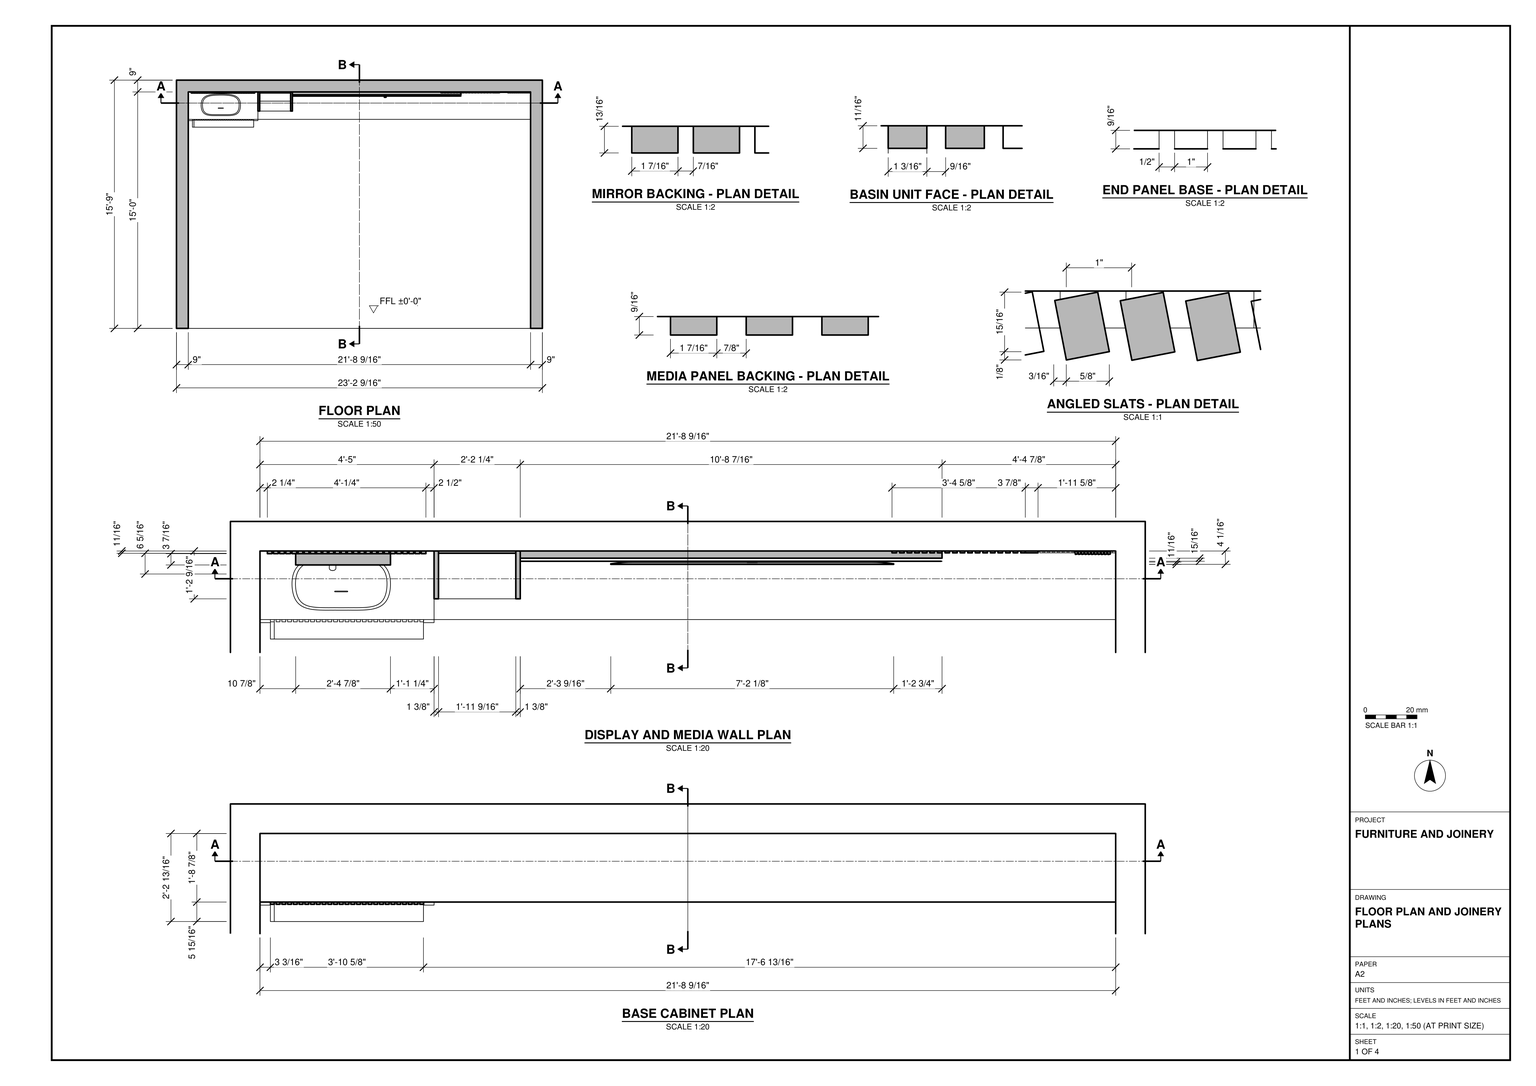
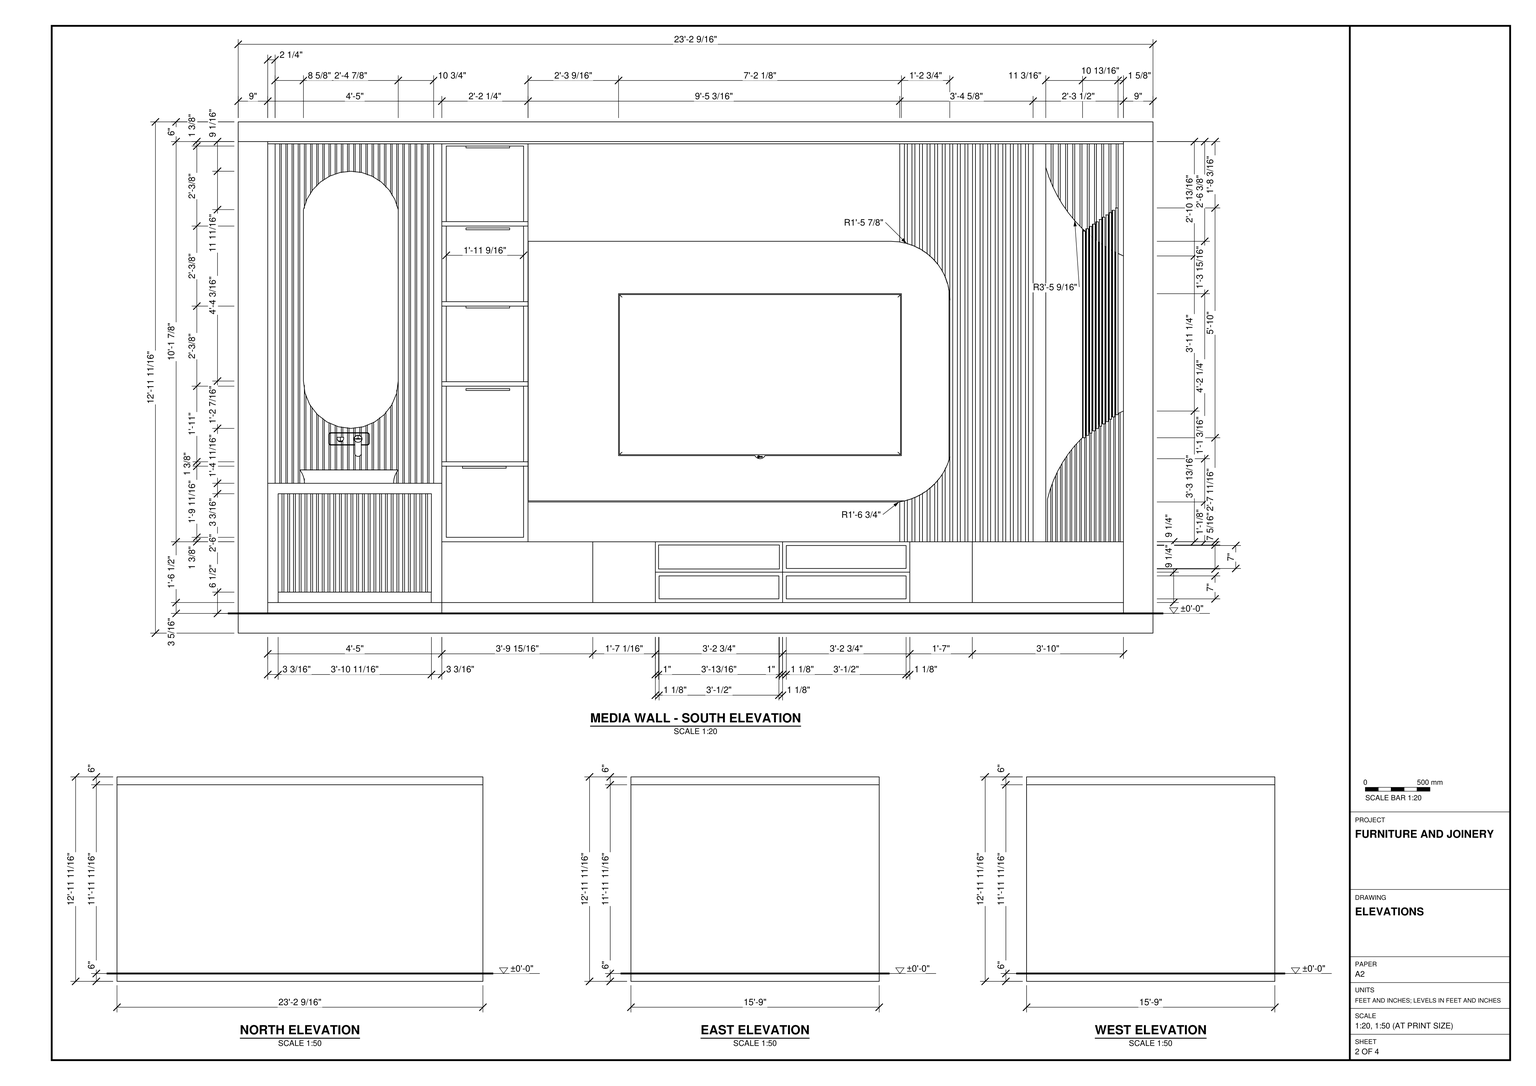
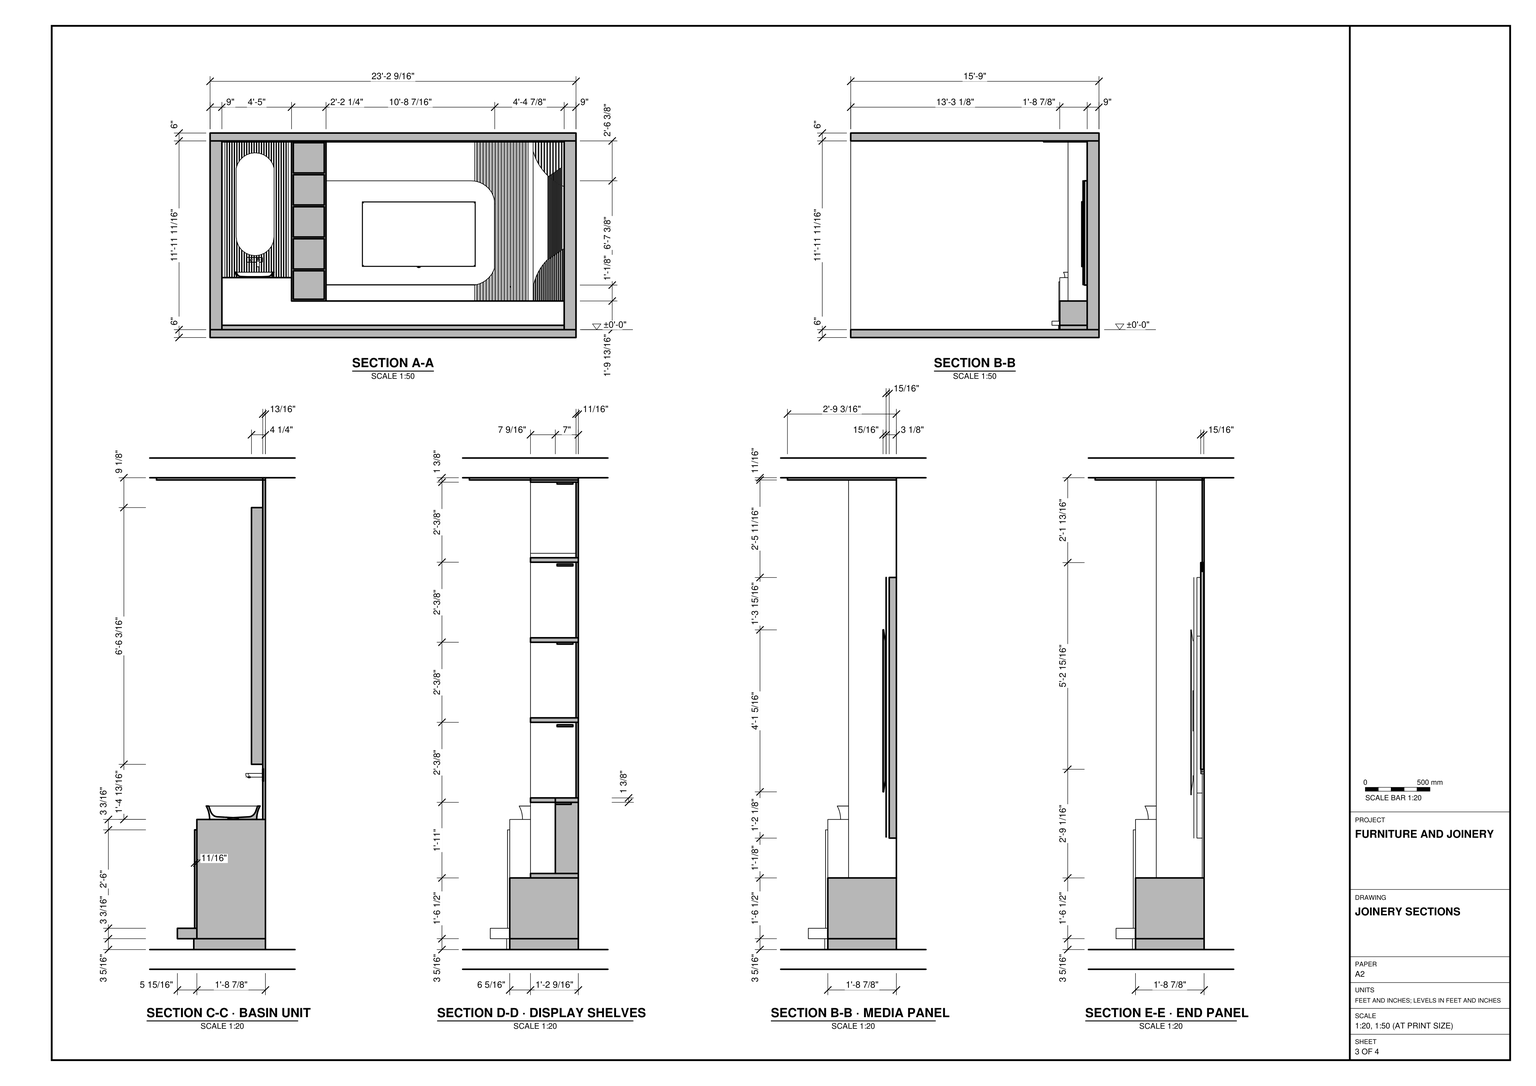
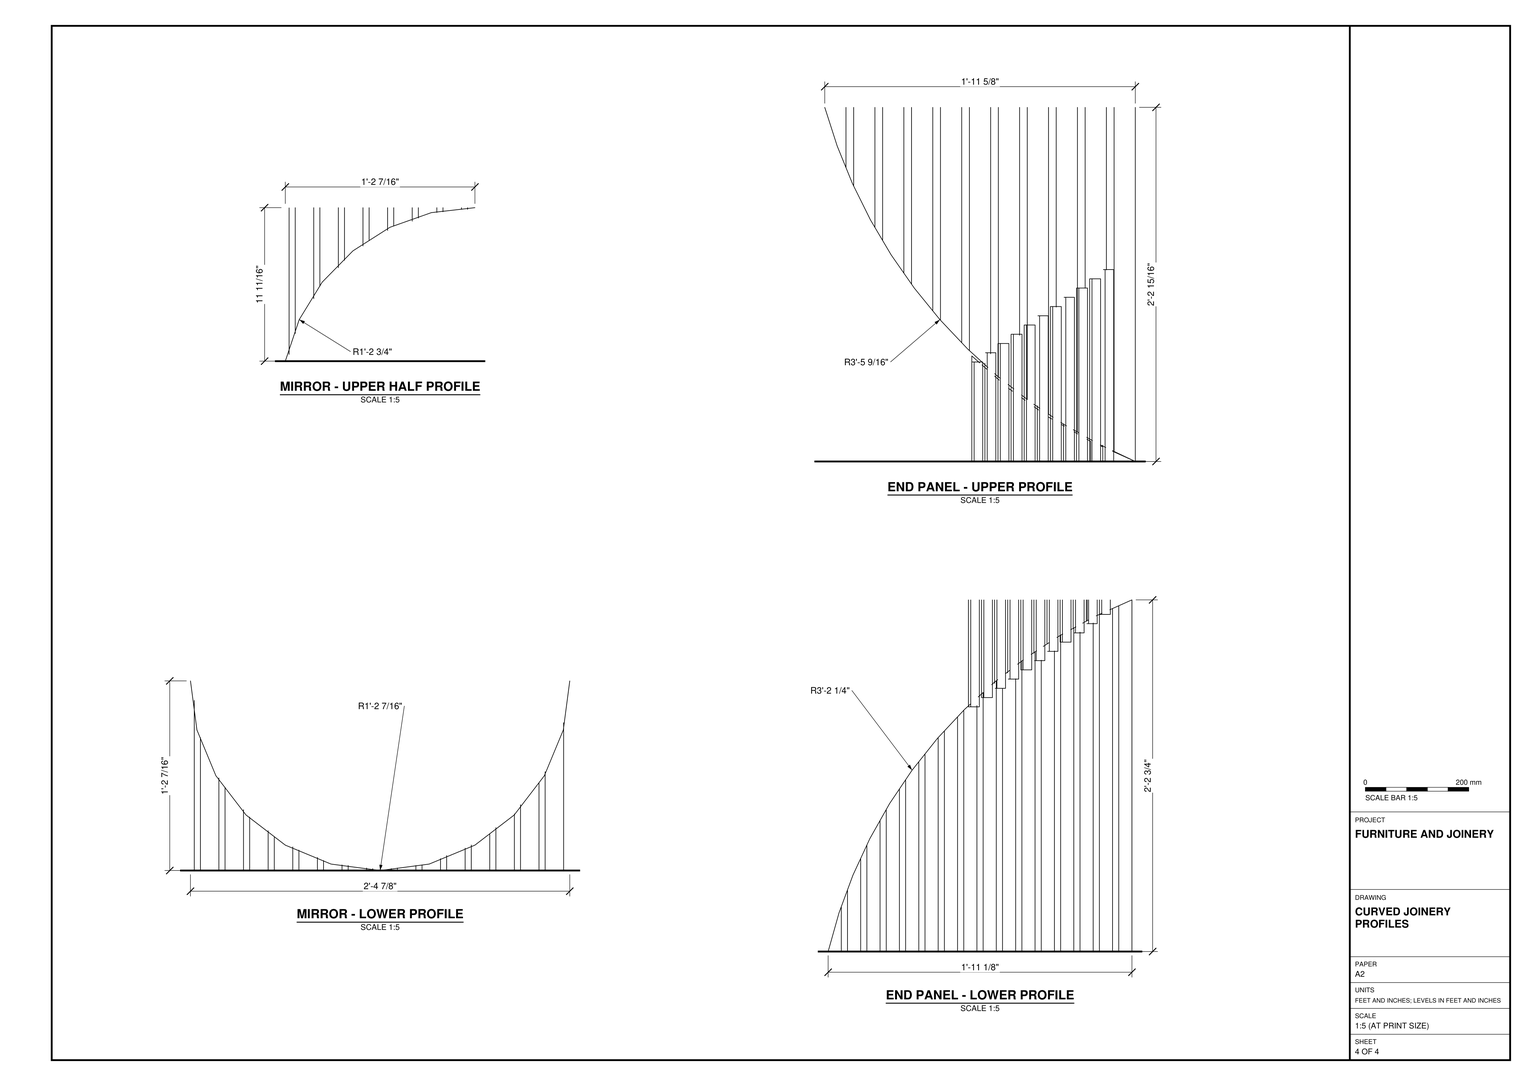
Build the wall-to-wall joinery and its room shell in SketchUp from task_files/diagram_01.pdf. Work in feet and inches. The overall model is 23'-2 9/16" wide, 15'-9" deep and 12'-11 11/16" high, with the finished floor at ±0'-0". Model the 9" rear wall and side returns between the 6" floor and overhead slabs. Leave the front open as shown in plan.

Use the south elevation to set out the joinery from left to right. Start with the ribbed basin cabinet, countertop basin and wall-mounted tap beneath a tall mirror with rounded ends. Set the mirror against vertical ribs. Fit the narrow stack of open display shelves between the basin bay and the media panel. Mount the screen on the broad panel, rounding the panel’s upper and lower right corners and leaving the ribbed backing visible beyond it. At the far right, follow the plan detail for the angled slats and the elevation for their curved termination.

Use the base cabinet plan and sections to set the cabinet depths, the projecting base at the basin and the setback of the display shelves. Match the arrangement of plain cabinet fronts and central framed openings below the screen. Decor and loose items may be any suitable library components. Keep each shell element and each joinery or furniture piece in a separate group or component, and use components for repeated parts. Save one SketchUp model as output_files/fitted_media_wall_with_basin_and_display_shelves.skp.

# SketchUp Ruby script. Lengths in inches.
U = 1.inch
M = Sketchup.active_model
def pt(a) = Geom::Point3d.new(a.map { |v| v * U })
def face(e, loops, mat)
  f = e.add_face(loops[0].map { |a| pt(a) })
  loops[1..].each { |l| e.add_face(l.map { |a| pt(a) }).erase! }
  f.material = f.back_material = mat if mat
  f
end
# faces: each face lists its corners as indices into pts; further lists are holes
def faces(e, pts, list, mat = nil) = list.each { |f| face(e, (f[0].is_a?(Array) ? f : [f]).map { |l| l.map { |i| pts[i] } }, mat) }
# xy, xz, yz: faces in a plane at the given z, y or x. An outline is a flat list of corners, or four numbers for a rectangle; further outlines are holes
def ring(l) = l.size == 4 ? [[l[0], l[1]], [l[2], l[1]], [l[2], l[3]], [l[0], l[3]]] : l.each_slice(2).to_a
def flat(e, list, mat, &to3) = list.each { |f| face(e, (f[0].is_a?(Array) ? f : [f]).map { |l| ring(l).map { |u, v| to3.(u, v) } }, mat) }
def xy(e, z, list, mat = nil) = flat(e, list, mat) { |x, y| [x, y, z] }
def xz(e, y, list, mat = nil) = flat(e, list, mat) { |x, z| [x, y, z] }
def yz(e, x, list, mat = nil) = flat(e, list, mat) { |y, z| [x, y, z] }
def lines(e, pts, list) = list.each { |a, b| e.add_line(pt(pts[a]), pt(pts[b])) }
# prism: a flat outline (further loops are holes) pulled along v
def prism(e, loops, v, mat = nil)
  f = face(e, loops, mat); d = Geom::Vector3d.new(v.map { |x| x * U })
  f.pushpull(f.normal.samedirection?(d) ? d.length : -d.length)
end
def box(e, o, s, mat = nil) = prism(e, [[o, [o[0] + s[0], o[1], o[2]], [o[0] + s[0], o[1] + s[1], o[2]], [o[0], o[1] + s[1], o[2]]]], [0, 0, s[2]], mat)
def at(x, y, z, deg = 0) = Geom::Transformation.translation(pt([x, y, z])) * Geom::Transformation.rotation(ORIGIN, Z_AXIS, deg.degrees)
def axes(o, x, y, z) = Geom::Transformation.new([*x, 0, *y, 0, *z, 0, *pt(o).to_a, 1])
def part(name) = M.definitions.add(name)
# library, detail: a bought-in or finely detailed component or shape, given as its bounding box
def library(name, o, s) = part(name).tap { |d| box(d.entities, o, s) }
def detail(e, o, s) = box(e.add_group.entities, o, s)
def put(e, d, t, mat = nil) = e.add_instance(d, t).tap { |i| i.material = mat if mat }
def group(e, t, mat = nil) = e.add_group.tap { |g| g.transformation = t; g.material = mat if mat }.entities
root = M.entities
M.materials.add("Gold 24k").color = [255, 235, 175]
M.materials.add("[Color E01]").color = [255, 255, 204]
M.materials.add("[Color M01]").color = [226, 226, 226]
M.materials.add("[Color M04]").color = [142, 142, 142]
M.materials.add("[Color_A04]").color = [219, 164, 177]
M.materials.add("[Square Glass Tile 02]").color = [120, 183, 140]
M.materials.add("[Tile Various Tan]").color = [214, 196, 169]
M.materials.add("[Wood Bamboo]").color = [177, 105, 43]
M.materials.add("bottom").color = [86, 95, 57]
M.materials.add("glass").color = [0, 0, 0]
M.materials.add("product_RG_W___dLorraine_80x80_Kepingan2").color = [228, 228, 223]
c1 = part("Component\#206")
xy(c1.entities,0,[[0,0,28.17,0,28.6,0.22,29.02,0.51,29.42,0.87,29.8,1.3,30.15,1.79,30.47,2.33,30.76,2.93,31.01,3.58,31.23,4.26,31.41,4.98,31.47,5.33,31.47,27.49,31.4,28.15,31.21,29.1,30.96,30,30.64,30.83,30.26,31.58,29.83,32.24,29.35,32.8,28.84,33.24,28.29,33.5625,27.73,33.76,27.16,33.82,0,33.82]],"product_RG_W___dLorraine_80x80_Kepingan2")
p = [[31.51,27.17,0],[31.55,26.17,0],[31.47,27.49,0],[31.55,5.73,0],[31.47,5.33,0],[28.17,0,0],
  [27.73,-0.15,0]]
lines(c1.entities,p,[[0,1],[2,0],[3,4],[5,6]])
c2 = library("Tv (1)",[0,2.0625,1.86],[28.07,0.6875,16.17])
c3 = library("plants",[135.36,200.5,-11.65],[19.49,26.19,113.21])
c4 = library("flowers",[56.72,269.05,39.62],[28.97,17.04,51.64])
c5 = library("vase2",[75.89,50.38,0],[14.78,14.14,22.97])
c6 = library("kohler - sink-and-tap",[15.05,116.22,-0.04],[21.62,17.39,12.15])
c7 = library("Knut",[-54.49,-63.02,-6.86],[166.1,126.59,175.47])
c8 = library("1935+Ford+Sedan+Toy+Car",[-0.69,-0.01,-0.125],[9.44,3.81,3.74])
c9 = library("Vase_Flowers_22.skp",[-5.3,-7.7,-1.52],[10.79,13.24,11.97])
c10 = part("stem")
p = [[8.92,1.38,83.34],[12.34,1.73,96.125],[8.32,0.48,83.4375],[8.19,2.35,83.4375],[11.85,2.6,96.21],[6.99,0.55,83.63],
  [10.86,0.86,96.39],[11.85,0.86,96.21],[6.86,2.43,83.63],[10.86,2.6,96.39],[6.26,1.53,83.73],[10.36,1.73,96.48],
  [16.61,1.73,120.56],[16.3,1.18,120.63],[16.3,2.28,120.63],[15.69,1.18,120.77],[15.69,2.28,120.77],[15.375,1.73,120.84],
  [21.36,1.47,144.07],[21.11,1.47,144.13],[21.49,1.6875,144.05],[21.36,1.91,144.07],[21.11,1.91,144.13],[20.99,1.6875,144.16]]
faces(c10.entities,p,[[0,1,2],[3,4,0],[1,0,4],[5,2,6],[7,2,1],[7,6,2],[8,9,3],[4,3,9],
  [5,6,10],[8,10,9],[11,10,6],[11,9,10],[7,1,12,13],[1,4,14,12],[7,13,15,6],[4,9,16,14],
  [6,15,17,11],[17,16,9,11],[18,19,15,13],[12,20,18,13],[20,12,14,21],[21,14,16,22],[19,23,17,15],[16,17,23,22]],"bottom")
faces(c10.entities,p,[[18,20,21,22,23,19]])
c11 = part("leaf\#1")
xy(c11.entities,0,[[1.27,0.625,0,1.89,0,3.7,1.27,5.43,3.34,6.6875,3.34,1.02]],"bottom")
p = [[3.34,6.6875,0],[5.69,5.05,-0.75],[6.53,3.7,-1.02],[6.53,1.64,-1.02],[4.9375,0.625,-0.51],[3.34,1.02,0],
  [3.34,0.4375,0],[3.34,0,0]]
faces(c11.entities,p,[[0,1,2,3,4,5]],"bottom")
lines(c11.entities,p,[[5,6],[6,7]])
c12 = part("petal\#1")
p = [[0.59,-0.98,-0.45],[0.74,-1.1,-0.29],[0.41,-0.67,-0.14],[0.42,-0.77,-0.38],[1.2,-1.19,-0.06],[0.54,-0.34,0.24],
  [1.12,0.01,0.5],[1.78,-0.84,0.21],[1.45,-0.41,0.36],[0,0.42,0],[0.09,0.28,0.2],[0.09,0.84,0.2],
  [0,0.7,0],[1.87,-0.35,0.24],[2.18,-0.15,0.17],[2.39,0.2,0.15],[2.22,0.41,0.23],[1.85,0.28,0.32],
  [1.6,0,0.36],[0.45,0,0.45],[0.45,1.12,0.45],[1.87,0.28,0.35],[1.87,0.84,0.35],[2.23,0.7,0.23],
  [1.51,0.33,0.48],[1.16,0.56,0.6],[1.16,0,0.6],[1.51,0.79,0.48],[1.16,1.12,0.6]]
faces(c12.entities,p,[[0,1,2,3],[1,4,5,2],[6,5,4,7,8],[9,10,11,12],[13,8,7,14],[14,15,16,17,18,8,13],[10,19,20,11],[21,16,22],
  [23,22,16],[6,8,18,17],[24,25,26,21],[22,27,25,24,21],[28,25,27,22],[28,20,19,26,25]],"[Color_A04]")
c13 = part("flower\#1")
put(c13.entities,c12,axes([2.1,0,0.625],[-0.03304,0.72958,0.14199],[-0.77918,0,-0.18132],[-0.17781,-0.15676,0.76408]))
put(c13.entities,c12,axes([3.38,2.1,1.25],[-0.77918,0,-0.18132],[0,-0.8,0],[-0.18132,0,0.77918]))
put(c13.entities,c12,axes([0.01,1.2,0],[0.7057,0,0.37681],[0,0.8,0],[-0.37681,0,0.7057]))
put(c13.entities,c12,axes([1.16,3.49,0.73],[0,-0.8,0],[0.77918,0,0.18132],[-0.18132,0,0.77918]))
c14 = part("Plant_flower")
p = [[4.13,-5.21,48.5625],[2.97,-5.27,48.18],[2.1,-5.33,47.33],[1.6875,-5.39,46.18],[2.87,-8.33,51.63],[2.46,-7.41,51.49],
  [2,-6.68,50.88],[1.58,-6.29,49.94]]
lines(c14.entities,p,[[0,1],[1,2],[2,3],[4,5],[6,7],[5,6]])
put(c14.entities,c10,axes([-0.85,0.55,-1.29],[0.10275,-0.38349,0],[0.38349,0.10275,0],[0,0,0.39701]))
put(c14.entities,c11,axes([3.82,-6.52,48.84],[0.09945,0.40738,-0.08753],[0.52591,-0.18667,-0.27125],[-0.22953,-0.03449,-0.42129]))
put(c14.entities,c13,axes([6.9,-4.04,53.68],[-2.40969,0.82543,0.59906],[-0.96837,-2.33406,-0.67913],[0.32013,-0.84712,2.45494]))
put(c14.entities,c11,axes([1.64,-8.47,52.18],[0.38389,0.04123,-0.17257],[-0.11872,-0.44244,-0.27916],[-0.18424,0.2028,-0.32786]))
c15 = part("stem2")
p = [[11.85,0.86,96.21],[12.34,1.73,96.125],[16.61,1.73,120.56],[16.3,1.18,120.63],[11.85,2.6,96.21],[16.3,2.28,120.63],
  [15.69,1.18,120.77],[10.86,0.86,96.39],[10.86,2.6,96.39],[15.69,2.28,120.77],[15.375,1.73,120.84],[10.36,1.73,96.48],
  [21.36,1.47,144.07],[21.11,1.47,144.13],[21.49,1.6875,144.05],[21.36,1.91,144.07],[21.11,1.91,144.13],[20.99,1.6875,144.16]]
faces(c15.entities,p,[[0,1,2,3],[1,4,5,2],[0,3,6,7],[4,8,9,5],[7,6,10,11],[10,9,8,11],[12,13,6,3],[2,14,12,3],
  [14,2,5,15],[15,5,9,16],[13,17,10,6],[9,10,17,16]],"bottom")
faces(c15.entities,p,[[12,14,15,16,17,13]])
c16 = part("Plant_flower2")
p = [[2.87,-8.33,51.63],[2.46,-7.41,51.49],[2,-6.68,50.88],[1.58,-6.29,49.94]]
lines(c16.entities,p,[[0,1],[2,3],[1,2]])
put(c16.entities,c15,axes([-0.85,0.55,-1.29],[0.10275,-0.38349,0],[0.38349,0.10275,0],[0,0,0.39701]))
put(c16.entities,c13,axes([6.9,-4.04,53.68],[-2.40969,0.82543,0.59906],[-0.96837,-2.33406,-0.67913],[0.32013,-0.84712,2.45494]))
put(c16.entities,c11,axes([1.64,-8.47,52.18],[0.38389,0.04123,-0.17257],[-0.11872,-0.44244,-0.27916],[-0.18424,0.2028,-0.32786]))
c17 = part("Vase_Quarter\#3")
xy(c17.entities,0,[[0,0,0,0.8,0.21,0.8,0.59,0.59,0.8,0.21,0.8,0]])
xz(c17.entities,0.78,[[0,9.66,0.21,10.84]])
yz(c17.entities,0.78,[[0,9.66,0.21,10.84]])
p = [[0.8,0,0],[0.8,0.21,0],[1.35,0.42,2.81],[1.35,0,2.81],[0.59,0.59,0],[1.01,1.01,2.81],
  [0.21,0.8,0],[0.42,1.35,2.81],[0,0.8,0],[0,1.35,2.81],[1.51,0.46,4.94],[1.51,0,4.94],
  [1.125,1.125,4.94],[0.46,1.51,4.94],[0,1.51,4.94],[1.43,0.43,6.19],[1.43,0,6.19],[1.07,1.07,6.19],
  [0.43,1.43,6.19],[0,1.43,6.19],[1,0.27,8.5],[1,0,8.5],[0.73,0.73,8.5],[0.27,1,8.5],
  [0,1,8.5],[0.78,0.21,9.66],[0.78,0,9.66],[0.57,0.57,9.66],[0.21,0.78,9.66],[0,0.78,9.66],
  [0.57,0.57,10.84],[0.78,0.21,10.84],[0.21,0.78,10.84],[1,0.27,12],[1,0,12],[0.78,0,10.84],
  [0.73,0.73,12],[0.27,1,12],[0,0.78,10.84],[0,1,12]]
faces(c17.entities,p,[[0,1,2,3],[4,5,2,1],[5,4,6,7],[7,6,8,9],[2,10,11,3],[5,12,10,2],[12,5,7,13],[13,7,9,14],
  [10,15,16,11],[12,17,15,10],[12,13,18,17],[13,14,19,18],[15,20,21,16],[17,22,20,15],[17,18,23,22],[18,19,24,23],
  [25,26,21,20],[22,27,25,20],[23,28,27,22],[23,24,29,28],[27,30,31,25],[28,32,30,27],[33,34,35,31],[30,36,33,31],
  [32,37,36,30],[32,38,39,37]])
c18 = part("vase_thin\#1")
put(c18.entities,c17,at(0,0,0))
put(c18.entities,c17,at(0,0,0,90))
put(c18.entities,c17,at(0,0,0,180))
put(c18.entities,c17,at(0,0,0,-90))
c19 = part("Flowers in vase")
put(c19.entities,c14,axes([3.625,2.02,-8.35],[-0.06695,-0.33202,0.02963],[0.33329,-0.0672,0],[0.00586,0.02905,0.33871]))
put(c19.entities,c14,axes([1.32,2.29,-9.75],[-0.088,0.32841,0],[-0.32841,-0.088,0],[0,0,0.34]))
put(c19.entities,c16,axes([3.73,4.01,-12],[0.14851,-0.30585,0],[0.30585,0.14851,0],[0,0,0.34]))
put(c19.entities,c18,axes([2.72,2.71,0],[1,0,0],[0,1,0],[0,0,0.44]))
put(c19.entities,c14,axes([2.75,3.98,-10.5],[0.33881,-0.02845,0],[0.02845,0.33881,0],[0,0,0.34]))
c20 = library("Boeket",[-0.32,-1.04,0],[21.7,21.08,20.36])
c21 = library("Standing figure",[0,25.9,1.53],[28.99,24.65,71.95])
c22 = part("Group\#64")
box(c22.entities,[0,0,-0.5625],[13.3125,4.8125,0.5625],"Gold 24k")
xz(root,180,[[12.66,39.625,59.52,143.6875]])
p = [[86.9,165.4375,117.96],[88.26,165.4375,117.96],[63.36,165.4375,117.96],[62.01,165.4375,117.96],[63.36,165.4375,93.58],[62.01,165.4375,93.58],
  [86.9,165.4375,93.58],[88.26,165.4375,93.58],[86.9,165.4375,44.83],[88.26,165.4375,44.83],[63.36,165.4375,44.83],[62.01,165.4375,44.83],
  [63.36,165.4375,69.21],[62.01,165.4375,69.21],[86.9,165.4375,69.21],[88.26,165.4375,69.21]]
lines(root,p,[[0,1],[2,3],[4,5],[6,7],[8,9],[10,11],[12,13],[14,15]])
put(root,c1,axes([88.32,176.875,34.28],[4.07098,0,0],[0,0,2.33687],[0,-1,0]))
put(root,c2,axes([115.82,173.87,41.33],[3.06877,0,0],[0,1,0],[0,0,3.10806]))
put(root,c3,at(-69.78,-51.48,34.56))
put(root,c4,at(-4.07,-109.27,0))
put(root,c5,axes([72.44,16.74,21.8125],[2.034,0,0],[0,2.5752,0],[0,0,2.21026]))
put(root,c6,axes([-2.125,45.76,39.68],[1.38691,0,0],[0,1,0],[0,0,1.27]))
put(root,c7,axes([72.5625,173.01,47.01],[0.10478,0,0],[0,0.12012,0],[0,0,0.11949]))
put(root,c8,axes([91.46,164.1875,22.125],[3.36837,-0.79021,0],[0.68519,2.9207,0],[0,0,3.48]))
put(root,c9,axes([74.93,169.72,95],[2.18099,0,0],[0,1.6698,0],[0,0,1.86]))
put(root,c19,axes([223.9,161.41,21.8125],[1.74,0,0],[0,1.9,0],[0,0,1.76045]))
put(root,c20,at(3.73,159.46,40.3125))
put(root,c21,at(13.82,101.37,0))
g1 = group(root,at(9,159.12,0))
xy(g1,0,[[0,-0.9375,0,20.88,260.5625,20.88,260.5625,0,53.01,0,53.01,-0.9375]])
xy(g1,3.3125,[[0,-0.9375,3.17,0],[3.17,-0.9375,49.78,0],[49.78,-0.9375,53.01,0],[0,0,260.5625,20.88]])
xy(g1,21.8125,[[53.01,0,260.5625,0,260.5625,20.88,79.26,20.88,79.26,6.32,53.01,6.32]])
xy(g1,39.625,[[0,0,53.01,20.88]])
xy(g1,119.3125,[[54.36,20.19,77.9,20.88]],"[Wood Bamboo]")
xy(g1,142.33,[[54.36,20.19,77.9,20.88]],"[Wood Bamboo]")
xz(g1,-0.9375,[[0,0,53.01,3.3125]],"[Color M01]")
xz(g1,0,[[53.01,0,260.5625,3.3125],[3.17,3.3125,49.78,6.48],[[118.03,3.3125,156.77,12.5625],[119.16,4.44,155.65,11.44]],[[156.77,3.3125,195.51,12.5625],[157.9,4.44,194.39,11.44]],[119.16,4.44,155.65,11.44],
  [157.9,4.44,194.39,11.44],[3.17,6.48,4.35,36.46],[4.35,6.48,49.84,36.46],[[118.03,12.5625,156.77,21.8125],[119.01,13.54,155.8,20.84]],[[156.77,12.5625,195.51,21.8125],[157.9,13.69,194.39,20.69]],
  [119.01,13.54,155.8,20.84],[157.9,13.69,194.39,20.69]])
xz(g1,0,[[0,3.3125,3.17,3.3125,3.17,36.46,49.84,36.46,49.84,6.48,49.78,6.48,49.78,3.3125,53.01,3.3125,53.01,39.625,0,39.625]],"[Color M01]")
xz(g1,0,[[53.01,3.3125,98.97,21.8125],[98.97,3.3125,118.03,21.8125],[195.51,3.3125,214.54,21.8125],[214.54,3.3125,260.5625,21.8125]],"[Color M04]")
xz(g1,20.88,[[0,0,260.5625,3.3125],[0,3.3125,0,39.625,53.01,39.625,53.01,21.8125,260.5625,21.8125,260.5625,3.3125]])
xz(g1,20.88,[[54.36,119.3125,77.9,142.33]],"[Wood Bamboo]")
yz(g1,0,[[-0.9375,0,20.88,3.3125],[0,3.3125,20.88,39.625]])
yz(g1,53.01,[[-0.9375,0,0,3.3125],[0,21.8125,20.88,39.625]])
yz(g1,54.36,[[20.19,119.3125,20.88,142.33]],"[Wood Bamboo]")
yz(g1,77.9,[[20.19,119.3125,20.88,142.33]],"[Wood Bamboo]")
yz(g1,260.5625,[[0,0,20.88,3.3125],[0,3.3125,20.88,21.8125]])
g2 = group(g1,at(3.17,0,6.48),"[Color M01]")
box(g2,[0,-0.6875,0],[1.18,0.6875,29.98])
box(g2,[1.75,-0.6875,0],[1.18,0.6875,29.98])
box(g2,[3.5,-0.6875,0],[1.18,0.6875,29.98])
box(g2,[5.25,-0.6875,0],[1.18,0.6875,29.98])
box(g2,[7,-0.6875,0],[1.18,0.6875,29.98])
box(g2,[8.75,-0.6875,0],[1.18,0.6875,29.98])
box(g2,[10.5,-0.6875,0],[1.18,0.6875,29.98])
box(g2,[12.25,-0.6875,0],[1.18,0.6875,29.98])
box(g2,[14,-0.6875,0],[1.17,0.6875,29.98])
box(g2,[15.75,-0.6875,0],[1.17,0.6875,29.98])
box(g2,[17.5,-0.6875,0],[1.17,0.6875,29.98])
box(g2,[19.25,-0.6875,0],[1.17,0.6875,29.98])
box(g2,[21,-0.6875,0],[1.17,0.6875,29.98])
box(g2,[22.75,-0.6875,0],[1.17,0.6875,29.98])
box(g2,[24.5,-0.6875,0],[1.17,0.6875,29.98])
box(g2,[26.25,-0.6875,0],[1.17,0.6875,29.98])
box(g2,[27.99,-0.6875,0],[1.18,0.6875,29.98])
box(g2,[29.74,-0.6875,0],[1.18,0.6875,29.98])
box(g2,[31.49,-0.6875,0],[1.18,0.6875,29.98])
box(g2,[33.24,-0.6875,0],[1.18,0.6875,29.98])
box(g2,[34.99,-0.6875,0],[1.18,0.6875,29.98])
box(g2,[36.74,-0.6875,0],[1.18,0.6875,29.98])
box(g2,[38.49,-0.6875,0],[1.18,0.6875,29.98])
box(g2,[40.24,-0.6875,0],[1.18,0.6875,29.98])
box(g2,[41.99,-0.6875,0],[1.18,0.6875,29.98])
box(g2,[43.74,-0.6875,0],[1.18,0.6875,29.98])
box(g2,[45.49,-0.6875,0],[1.18,0.6875,29.98])
g3 = group(g1,at(3.17,0,3.3125),"[Color E01]")
prism(g3,[[[46.61,0,0],[0,0,0],[0,0,3.17],[1.18,0,3.17],[46.61,0,3.17]]],[0,-5.9375,0])
g4 = group(g1,at(53.01,6.32,21.8125),"[Wood Bamboo]")
xy(g4,0,[[0,0,26.25,14.5625]])
xy(g4,1.36,[[1.36,0,24.89,14.5625]])
xy(g4,23.02,[[1.36,0,24.89,14.5625]])
xy(g4,24.375,[[1.36,0,24.89,14.5625]])
xy(g4,47.39,[[1.36,0,24.89,14.5625]])
xy(g4,48.75,[[1.36,0,24.89,14.5625]])
xy(g4,71.77,[[1.36,0,24.89,14.5625]])
xy(g4,73.125,[[1.36,0,24.89,14.5625]])
xy(g4,96.14,[[1.36,0,24.89,14.5625]])
xy(g4,97.5,[[1.36,0,24.89,14.5625]])
xy(g4,120.52,[[1.36,0,24.89,14.5625]])
xy(g4,121.875,[[0,0,26.25,14.5625]])
xz(g4,0,[[[0,0,26.25,24.375],[1.36,1.36,24.89,23.02]],[0,24.375,1.36,24.375,1.36,47.39,24.89,47.39,24.89,24.375,26.25,24.375,26.25,48.75,0,48.75],[0,48.75,1.36,48.75,1.36,71.77,24.89,71.77,24.89,48.75,26.25,48.75,26.25,73.125,0,73.125],[0,73.125,1.36,73.125,1.36,96.14,24.89,96.14,24.89,73.125,26.25,73.125,26.25,97.5,0,97.5],[0,97.5,1.36,97.5,1.36,120.52,24.89,120.52,24.89,97.5,26.25,97.5,26.25,121.875,0,121.875]])
xz(g4,14.5625,[[[0,0,26.25,121.875],[1.36,24.375,24.89,47.39],[1.36,48.75,24.89,71.77],[1.36,73.125,24.89,96.14],[1.36,97.5,24.89,120.52],[1.36,1.36,24.89,23.02]]])
yz(g4,0,[[0,0,14.5625,121.875]])
yz(g4,1.36,[[0,1.36,14.5625,23.02],[0,24.375,14.5625,47.39],[0,48.75,14.5625,71.77],[0,73.125,14.5625,96.14],[0,97.5,14.5625,98.86],
  [0,98.86,14.5625,120.52]])
yz(g4,24.89,[[0,1.36,14.5625,23.02],[0,24.375,14.5625,47.39],[0,48.75,14.5625,71.77],[0,73.125,14.5625,96.14],[0,97.5,14.5625,98.86],
  [0,98.86,14.5625,120.52]])
yz(g4,26.25,[[0,0,14.5625,121.875]])
g5 = group(g1,at(54.36,20.19,119.3125))
xz(g5,-6.32,[[0,-96.14,23.54,-73.125]],"[Wood Bamboo]")
xz(g5,0,[[0,-73.125,23.54,-50.11],[0,-48.75,23.54,-25.73],[0,-24.375,23.54,-1.36],[0,0,23.54,23.02]],"[Wood Bamboo]")
put(g1,c22,at(60.36,14.41,142.33))
put(g1,c22,at(60.36,14.41,117.39))
put(g1,c22,at(60.36,14.41,93.58))
put(g1,c22,at(60.36,14.41,68.46))
put(g1,c22,at(59.28,13.875,44.78))
g6 = group(root,at(0,0,-6),"[Color M01]")
box(g6,[0,0,149.6875],[278.5625,189,6])
xy(g6,0,[[0,0,278.5625,189]],"[Square Glass Tile 02]")
xy(g6,6,[[0,0,278.5625,189]],"[Tile Various Tan]")
xz(g6,0,[[0,0,278.5625,6]],"[Color M01]")
xz(g6,189,[[0,0,278.5625,6]],"[Square Glass Tile 02]")
yz(g6,0,[[0,0,189,6]],"[Square Glass Tile 02]")
yz(g6,278.5625,[[0,0,189,6]],"[Square Glass Tile 02]")
g7 = group(g6,at(269.5625,169.89,149.6875))
xy(g7,-0.6875,[[-260.5625,-23.0625,0,10.11]],"[Color M01]")
xy(g7,0,[[-260.5625,-23.0625,0,10.11]])
xz(g7,-23.0625,[[-260.5625,-0.6875,0,0]],"[Color M01]")
xz(g7,10.11,[[-260.5625,-0.6875,0,0]])
yz(g7,-260.5625,[[-23.0625,-0.6875,10.11,0]])
yz(g7,0,[[-23.0625,-0.6875,10.11,0]])
g8 = group(root,at(11.25,180,39.625),"[Wood Bamboo]")
box(g8,[0,-0.8125,0],[1.41,0.8125,104.0625])
box(g8,[1.875,-0.8125,0],[1.4,0.8125,104.0625])
box(g8,[3.75,-0.8125,0],[1.41,0.8125,104.0625])
box(g8,[5.625,-0.8125,0],[1.41,0.8125,104.0625])
box(g8,[7.5,-0.8125,0],[1.4,0.8125,104.0625])
box(g8,[9.37,-0.8125,0],[1.41,0.8125,104.0625])
box(g8,[11.25,-0.8125,0],[1.4,0.8125,104.0625])
box(g8,[13.12,-0.8125,0],[1.41,0.8125,104.0625])
box(g8,[15,-0.8125,0],[1.4,0.8125,104.0625])
box(g8,[16.87,-0.8125,0],[1.41,0.8125,104.0625])
box(g8,[18.74,-0.8125,0],[1.41,0.8125,104.0625])
box(g8,[20.62,-0.8125,0],[1.41,0.8125,104.0625])
box(g8,[22.49,-0.8125,0],[1.41,0.8125,104.0625])
box(g8,[24.37,-0.8125,0],[1.41,0.8125,104.0625])
box(g8,[26.24,-0.8125,0],[1.41,0.8125,104.0625])
box(g8,[28.12,-0.8125,0],[1.4,0.8125,104.0625])
box(g8,[29.99,-0.8125,0],[1.41,0.8125,104.0625])
box(g8,[31.87,-0.8125,0],[1.4,0.8125,104.0625])
box(g8,[33.74,-0.8125,0],[1.41,0.8125,104.0625])
box(g8,[35.62,-0.8125,0],[1.4,0.8125,104.0625])
box(g8,[37.49,-0.8125,0],[1.41,0.8125,104.0625])
box(g8,[39.36,-0.8125,0],[1.41,0.8125,104.0625])
box(g8,[41.24,-0.8125,0],[1.41,0.8125,104.0625])
box(g8,[43.11,-0.8125,0],[1.41,0.8125,104.0625])
box(g8,[44.99,-0.8125,0],[1.4,0.8125,104.0625])
box(g8,[46.86,-0.8125,0],[1.41,0.8125,104.0625])
g9 = group(root,at(26.99,179.1875,70.78))
xz(g9,-3.4375,[[7.3125,-14.4375,11.05,-13.95,14.53,-12.5,17.52,-10.21,19.82,-7.22,21.26,-3.74,21.75,0,21.75,52.1875,20.6875,55.36,18.94,58.2,16.6,60.59,13.78,62.38,10.63,63.5,7.3125,63.875,3.99,63.5,0.84,62.38,-1.98,60.59,-4.32,58.2,-6.0625,55.36,-7.125,52.1875,-7.125,0,-6.63,-3.74,-5.19,-7.22,-2.9,-10.21,0.09,-12.5,3.58,-13.95]],"glass")
xz(g9,0,[[7.3125,-14.4375,3.58,-13.95,0.09,-12.5,-2.9,-10.21,-5.19,-7.22,-6.63,-3.74,-7.125,0,-7.125,52.1875,-6.0625,55.36,-4.32,58.2,-1.98,60.59,0.84,62.38,3.99,63.5,7.3125,63.875,10.63,63.5,13.78,62.38,16.6,60.59,18.94,58.2,20.6875,55.36,21.75,52.1875,21.75,0,21.26,-3.74,19.82,-7.22,17.52,-10.21,14.53,-12.5,11.05,-13.95]])
yz(g9,-7.125,[[-3.4375,0,0,52.1875]])
yz(g9,21.75,[[-3.4375,0,0,52.1875]])
p = [[3.58,0,-13.95],[7.3125,0,-14.4375],[7.3125,-3.4375,-14.4375],[3.58,-3.4375,-13.95],[11.05,0,-13.95],[11.05,-3.4375,-13.95],
  [0.09,0,-12.5],[0.09,-3.4375,-12.5],[14.53,0,-12.5],[14.53,-3.4375,-12.5],[-2.9,0,-10.21],[-2.9,-3.4375,-10.21],
  [17.52,0,-10.21],[17.52,-3.4375,-10.21],[-5.19,0,-7.22],[-5.19,-3.4375,-7.22],[19.82,0,-7.22],[19.82,-3.4375,-7.22],
  [-6.63,0,-3.74],[-6.63,-3.4375,-3.74],[21.26,0,-3.74],[21.26,-3.4375,-3.74],[-7.125,0,0],[-7.125,-3.4375,0],
  [21.75,0,0],[21.75,-3.4375,0],[-6.0625,0,55.36],[-7.125,0,52.1875],[-7.125,-3.4375,52.1875],[-6.0625,-3.4375,55.36],
  [21.75,0,52.1875],[20.6875,0,55.36],[20.6875,-3.4375,55.36],[21.75,-3.4375,52.1875],[-4.32,0,58.2],[-4.32,-3.4375,58.2],
  [18.94,0,58.2],[18.94,-3.4375,58.2],[-1.98,0,60.59],[-1.98,-3.4375,60.59],[16.6,0,60.59],[16.6,-3.4375,60.59],
  [0.84,0,62.38],[0.84,-3.4375,62.38],[13.78,0,62.38],[13.78,-3.4375,62.38],[3.99,0,63.5],[3.99,-3.4375,63.5],
  [10.63,0,63.5],[10.63,-3.4375,63.5],[7.3125,0,63.875],[7.3125,-3.4375,63.875]]
faces(g9,p,[[0,1,2,3],[1,4,5,2],[6,0,3,7],[4,8,9,5],[10,6,7,11],[8,12,13,9],[14,10,11,15],[12,16,17,13],
  [18,14,15,19],[16,20,21,17],[22,18,19,23],[20,24,25,21],[26,27,28,29],[30,31,32,33],[34,26,29,35],[31,36,37,32],
  [38,34,35,39],[36,40,41,37],[42,38,39,43],[40,44,45,41],[46,42,43,47],[44,48,49,45],[50,46,47,51],[48,50,51,49]])
g10 = group(root,at(0,0,0))
xy(g10,0,[[0,0,0,189,278.5625,189,278.5625,0,269.5625,0,269.5625,180,9,180,9,0]])
xy(g10,143.6875,[[0,0,9,0,9,180,269.5625,180,269.5625,0,278.5625,0,278.5625,189,0,189]])
xz(g10,0,[[0,0,9,143.6875],[269.5625,0,278.5625,143.6875]])
xz(g10,180,[[9,0,269.5625,143.6875]],"[Color E01]")
xz(g10,189,[[0,0,278.5625,143.6875]])
yz(g10,0,[[0,0,189,143.6875]])
yz(g10,9,[[0,0,180,143.6875]])
yz(g10,269.5625,[[0,0,180,143.6875]])
yz(g10,278.5625,[[0,0,189,143.6875]])
p = [[257.12,179.87,116.9],[259.91,179.91,114.43],[262.93,179.95,112.25],[266.16,179.98,110.39],[269.5625,180,108.86],[266.16,179.98,59.63],
  [257.12,179.87,116.4375],[257.12,179.87,53.49],[257.12,179.87,51.74]]
lines(g10,p,[[0,1],[1,2],[2,3],[3,4],[3,5],[0,6],[7,8]])
g11 = group(g10,at(88.26,180,33.94))
prism(g11,[[[112.89,0,0],[0,0,0],[0,0,79.375],[110.56,0,79.375],[112.89,0,79.22],[115.18,0,78.77],[117.4,0,78.01],[119.49,0,76.98],[121.4375,0,75.68],[123.2,0,74.14],[124.74,0,72.38],[126.04,0,70.4375],[127.07,0,68.34],[127.82,0,66.13],[128.28,0,63.83],[128.43,0,61.5],[128.43,0,13.72],[127.87,0,11.98],[127.15,0,10.3],[126.26,0,8.7],[125.22,0,7.19],[124.04,0,5.8],[122.73,0,4.52],[121.3,0,3.375],[119.77,0,2.38],[118.14,0,1.53],[116.45,0,0.85],[114.6875,0,0.34]]],[0,-2.1875,0])
g12 = group(g10,at(201.45,180,21.8125),"[Wood Bamboo]")
box(g12,[0,-0.5625,0],[1.41,0.5625,121.875])
box(g12,[2.31,-0.5625,0],[1.41,0.5625,121.875])
box(g12,[4.61,-0.5625,0],[1.41,0.5625,121.875])
box(g12,[6.92,-0.5625,0],[1.41,0.5625,121.875])
box(g12,[9.22,-0.5625,0],[1.41,0.5625,121.875])
box(g12,[11.53,-0.5625,0],[1.41,0.5625,121.875])
box(g12,[13.83,-0.5625,0],[1.41,0.5625,121.875])
box(g12,[16.14,-0.5625,0],[1.41,0.5625,121.875])
box(g12,[18.44,-0.5625,0],[1.41,0.5625,121.875])
box(g12,[20.75,-0.5625,0],[1.41,0.5625,121.875])
box(g12,[23.05,-0.5625,0],[1.41,0.5625,121.875])
box(g12,[25.36,-0.5625,0],[1.41,0.5625,121.875])
box(g12,[27.66,-0.5625,0],[1.41,0.5625,121.875])
box(g12,[29.97,-0.5625,0],[1.41,0.5625,121.875])
box(g12,[32.27,-0.5625,0],[1.41,0.5625,121.875])
box(g12,[34.58,-0.5625,0],[1.41,0.5625,121.875])
box(g12,[36.88,-0.5625,0],[1.41,0.5625,121.875])
box(g12,[39.1875,-0.5625,0],[1.41,0.5625,121.875])
g13 = group(g10,at(242.05,180,21.8125),"Gold 24k")
box(g13,[0,-0.5625,0],[3.87,0.5625,121.875],"Gold 24k")
g14 = group(g10,at(245.92,180,108.86),"[Wood Bamboo]")
xy(g14,34.82,[[0,-0.5625,1.62,0],[2.2,-0.5625,3.82,0],[4.41,-0.5625,6.02,0],[6.61,-0.5625,8.22,0],[8.81,-0.5625,10.43,0],
  [11.01,-0.5625,12.63,0],[13.22,-0.5625,14.83,0],[15.42,-0.5625,17.03,0],[17.62,-0.5625,19.24,0],[19.82,-0.5625,21.44,0],
  [22.03,-0.5625,23.64,0]])
xz(g14,-0.5625,[[23.64,0,23.64,34.82,22.03,34.82,22.03,0.77],[21.44,1.04,21.44,34.82,19.82,34.82,19.82,1.91,20.85,1.32],[19.24,2.24,19.24,34.82,17.62,34.82,17.62,3.21,18.17,2.85],[17.03,3.61,17.03,34.82,15.42,34.82,15.42,4.71,15.6,4.57],[14.83,5.17,14.83,34.82,13.22,34.82,13.22,6.4375],
  [12.63,6.97,12.63,34.82,11.01,34.82,11.01,8.44],[10.43,9.04,10.43,34.82,8.81,34.82,8.81,10.76],[8.22,11.47,8.22,34.82,6.61,34.82,6.61,13.5,6.82,13.2],[6.02,14.34,6.02,34.82,4.41,34.82,4.41,16.83,5.05,15.73],[3.82,17.82,3.82,34.82,2.2,34.82,2.2,20.97,3.48,18.39],
  [1.62,22.37,1.62,34.82,0,34.82,0,26.96,0.95,24.02]])
yz(g14,23.64,[[-0.5625,0,0,34.82]])
p = [[0,0,0],[0,-0.5625,0],[13.17,-0.5625,6.47],[12.63,-0.5625,6.97],[10.89,-0.5625,8.56],[10.43,-0.5625,9.04],
  [8.77,-0.5625,10.8],[8.22,-0.5625,11.47],[2.11,-0.5625,21.16],[1.62,-0.5625,22.37],[22.03,-0.5625,0.77],[21.44,-0.5625,1.04],
  [19.82,-0.5625,1.91],[19.24,-0.5625,2.24],[17.62,-0.5625,3.21],[17.03,-0.5625,3.61],[13.22,-0.5625,6.4375],[15.42,-0.5625,4.71],
  [14.83,-0.5625,5.17],[11.01,-0.5625,8.44],[8.81,-0.5625,10.76],[6.61,-0.5625,13.5],[6.02,-0.5625,14.34],[4.41,-0.5625,16.83],
  [3.82,-0.5625,17.82],[2.2,-0.5625,20.97]]
lines(g14,p,[[0,1],[2,3],[4,5],[6,7],[8,9],[10,11],[12,13],[14,15],[16,2],[17,18],[19,4],[20,6],
  [21,22],[23,24],[25,8]])
g15 = group(g10,at(268.56,180,21.8125),"[Wood Bamboo]")
xy(g15,0,[[-22.125,-0.5625,-21.12,0],[-20.65,-0.5625,-19.65,0],[-19.18,-0.5625,-18.17,0],[-17.7,-0.5625,-16.7,0],[-16.23,-0.5625,-15.22,0],
  [-14.75,-0.5625,-13.75,0],[-13.27,-0.5625,-12.27,0],[-11.8,-0.5625,-10.8,0],[-10.32,-0.5625,-9.32,0],[-8.85,-0.5625,-7.85,0],
  [-7.375,-0.5625,-6.37,0],[-5.9,-0.5625,-4.9,0],[-4.43,-0.5625,-3.42,0],[-2.95,-0.5625,-1.95,0],[-1.48,-0.5625,-0.47,0],
  [0,-0.5625,1,0]])
xz(g15,-0.5625,[[-22.125,0,-21.12,0,-21.12,16.47,-21.3,16,-22.125,13.05],[-20.65,0,-19.65,0,-19.65,20.14,-20.23,18.87,-20.65,17.75],[-19.18,0,-18.17,0,-18.17,23.03,-18.95,21.65,-19.18,21.16],[-17.7,0,-16.7,0,-16.7,25.43,-17.44,24.32,-17.7,23.86],[-16.23,0,-15.22,0,-15.22,27.5,-15.73,26.86,-16.23,26.13],
  [-14.75,0,-13.75,0,-13.75,29.34,-13.82,29.25,-14.75,28.09],[-13.27,0,-12.27,0,-12.27,30.91,-13.27,29.84],[-11.8,0,-10.8,0,-10.8,32.34,-11.73,31.49,-11.8,31.42],[-10.32,0,-9.32,0,-9.32,33.66,-9.47,33.55,-10.32,32.77],[-8.85,0,-7.85,0,-7.85,34.81,-8.85,34.03],
  [-7.375,0,-6.37,0,-6.37,35.87,-7.05,35.43,-7.375,35.17],[-5.9,0,-4.9,0,-4.9,36.83,-5.9,36.18],[-4.43,0,-3.42,0,-3.42,37.68,-4.43,37.14],[-2.95,0,-1.95,0,-1.95,38.49,-2.95,37.94],[-1.48,0,-0.47,0,-0.47,39.16,-1.48,38.71],
  [0,0,1,0,1,39.82,0,39.37]])
yz(g15,1,[[-0.5625,0,0,39.82]])
p = [[-11.8,0,39.82],[-11.8,-0.5625,39.82],[-1.79,-0.5625,38.57],[-1.95,-0.5625,38.49],[-1.48,-0.5625,38.71],[0,-0.5625,39.37],
  [-0.47,-0.5625,39.16],[-2.95,-0.5625,37.94],[-3.42,-0.5625,37.68],[-5.9,-0.5625,36.18],[-6.37,-0.5625,35.87],[-8.85,-0.5625,34.03],
  [-9.32,-0.5625,33.66],[-7.375,-0.5625,35.17],[-7.85,-0.5625,34.81],[-10.32,-0.5625,32.77],[-10.8,-0.5625,32.34],[-13.27,-0.5625,29.84],
  [-13.75,-0.5625,29.34],[-11.8,-0.5625,31.42],[-12.27,-0.5625,30.91],[-14.75,-0.5625,28.09],[-15.22,-0.5625,27.5],[-16.23,-0.5625,26.13],
  [-16.7,-0.5625,25.43],[-17.7,-0.5625,23.86],[-18.17,-0.5625,23.03],[-19.18,-0.5625,21.16],[-19.65,-0.5625,20.14],[-20.65,-0.5625,17.75],
  [-21.12,-0.5625,16.47],[-4.43,-0.5625,37.14],[-4.48,-0.5625,37.1],[-4.9,-0.5625,36.83]]
lines(g15,p,[[0,1],[2,3],[4,2],[5,6],[7,8],[9,10],[11,12],[13,14],[15,16],[17,18],[19,20],[21,22],
  [23,24],[25,26],[27,28],[29,30],[31,32],[32,33]])
g16 = group(g10,at(257.12,179.87,53.49),"[Wood Bamboo]")
prism(g16,[[[0,0,0],[0.65,0.13,0],[0.83,-0.78,0],[0.18,-0.91,0]]],[0,0,62.95])
prism(g16,[[[1,0,0.7],[1.65,0.125,0.7],[1.83,-0.78,0.7],[1.17,-0.91,0.7]]],[0,0,62.95])
prism(g16,[[[1.99,-0.01,1.41],[2.65,0.12,1.41],[2.82,-0.79,1.41],[2.17,-0.91,1.41]]],[0,0,62.95])
prism(g16,[[[2.99,-0.01,2.11],[3.65,0.12,2.11],[3.82,-0.79,2.11],[3.17,-0.92,2.11]]],[0,0,62.95])
prism(g16,[[[3.99,-0.02,2.8125],[4.64,0.11,2.8125],[4.82,-0.8,2.8125],[4.16,-0.92,2.8125]]],[0,0,62.95])
prism(g16,[[[4.98,-0.02,3.52],[5.64,0.11,3.52],[5.82,-0.8,3.52],[5.16,-0.93,3.52]]],[0,0,62.95])
prism(g16,[[[5.98,-0.02,4.22],[6.64,0.1,4.22],[6.8125,-0.8,4.22],[6.16,-0.93,4.22]]],[0,0,62.95])
prism(g16,[[[6.98,-0.03,4.92],[7.63,0.1,4.92],[7.81,-0.81,4.92],[7.16,-0.93,4.92]]],[0,0,62.95])
prism(g16,[[[7.98,-0.03,5.63],[8.63,0.09,5.63],[8.81,-0.8125,5.63],[8.15,-0.9375,5.63]]],[0,0,62.95])
prism(g16,[[[8.97,-0.04,6.33],[9.625,0.09,6.33],[9.8,-0.82,6.33],[9.15,-0.94,6.33]]],[0,0,62.95])
prism(g16,[[[9.97,-0.04,7.03],[10.625,0.09,7.03],[10.8,-0.82,7.03],[10.15,-0.95,7.03]]],[0,0,62.95])
